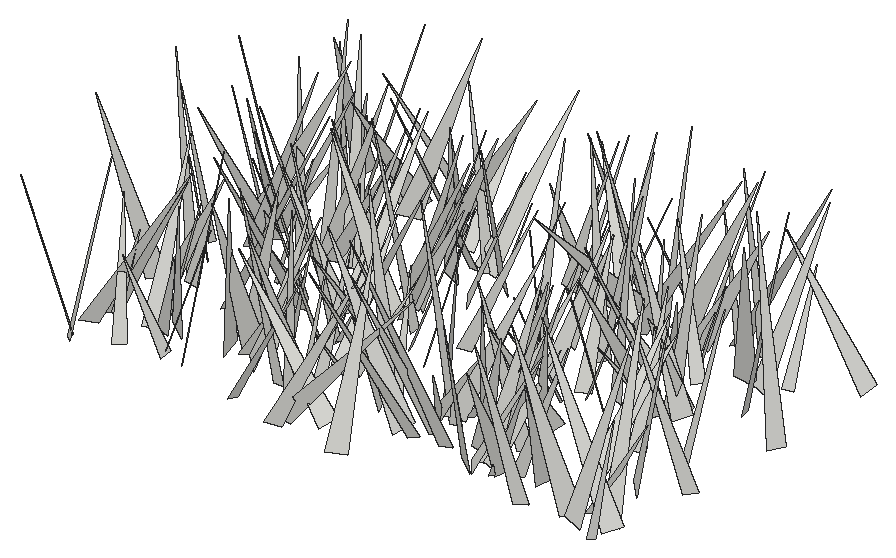
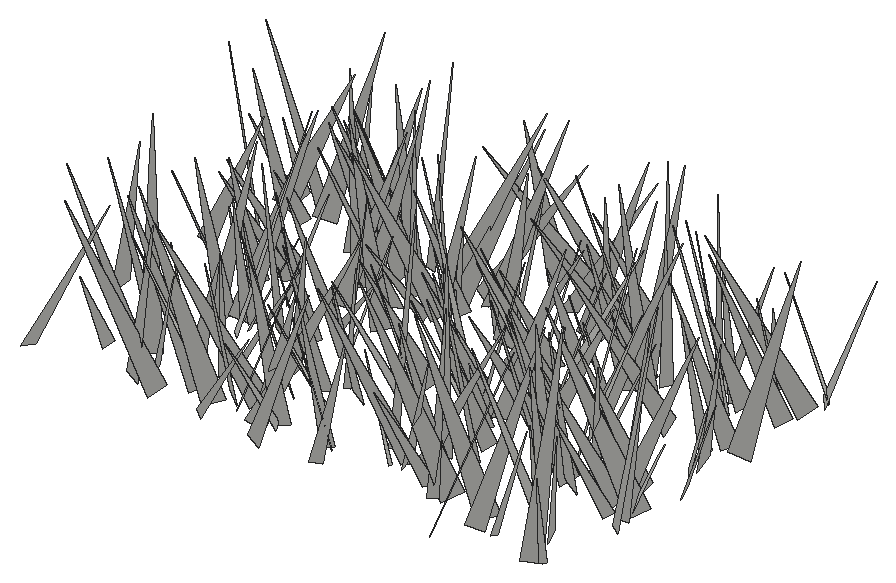
# SketchUp Ruby script. Lengths in inches.
U = 1.inch
M = Sketchup.active_model
def pt(a) = Geom::Point3d.new(a.map { |v| v * U })
def face(e, loops, mat)
  f = e.add_face(loops[0].map { |a| pt(a) })
  loops[1..].each { |l| e.add_face(l.map { |a| pt(a) }).erase! }
  f.material = f.back_material = mat if mat
  f
end
# faces: each face lists its corners as indices into pts; further lists are holes
def faces(e, pts, list, mat = nil) = list.each { |f| face(e, (f[0].is_a?(Array) ? f : [f]).map { |l| l.map { |i| pts[i] } }, mat) }
# xy, xz, yz: faces in a plane at the given z, y or x. An outline is a flat list of corners, or four numbers for a rectangle; further outlines are holes
def ring(l) = l.size == 4 ? [[l[0], l[1]], [l[2], l[1]], [l[2], l[3]], [l[0], l[3]]] : l.each_slice(2).to_a
def flat(e, list, mat, &to3) = list.each { |f| face(e, (f[0].is_a?(Array) ? f : [f]).map { |l| ring(l).map { |u, v| to3.(u, v) } }, mat) }
def xy(e, z, list, mat = nil) = flat(e, list, mat) { |x, y| [x, y, z] }
def xz(e, y, list, mat = nil) = flat(e, list, mat) { |x, z| [x, y, z] }
def yz(e, x, list, mat = nil) = flat(e, list, mat) { |y, z| [x, y, z] }
def lines(e, pts, list) = list.each { |a, b| e.add_line(pt(pts[a]), pt(pts[b])) }
# prism: a flat outline (further loops are holes) pulled along v
def prism(e, loops, v, mat = nil)
  f = face(e, loops, mat); d = Geom::Vector3d.new(v.map { |x| x * U })
  f.pushpull(f.normal.samedirection?(d) ? d.length : -d.length)
end
def box(e, o, s, mat = nil) = prism(e, [[o, [o[0] + s[0], o[1], o[2]], [o[0] + s[0], o[1] + s[1], o[2]], [o[0], o[1] + s[1], o[2]]]], [0, 0, s[2]], mat)
def at(x, y, z, deg = 0) = Geom::Transformation.translation(pt([x, y, z])) * Geom::Transformation.rotation(ORIGIN, Z_AXIS, deg.degrees)
def axes(o, x, y, z) = Geom::Transformation.new([*x, 0, *y, 0, *z, 0, *pt(o).to_a, 1])
def part(name) = M.definitions.add(name)
# library, detail: a bought-in or finely detailed component or shape, given as its bounding box
def library(name, o, s) = part(name).tap { |d| box(d.entities, o, s) }
def detail(e, o, s) = box(e.add_group.entities, o, s)
def put(e, d, t, mat = nil) = e.add_instance(d, t).tap { |i| i.material = mat if mat }
def group(e, t, mat = nil) = e.add_group.tap { |g| g.transformation = t; g.material = mat if mat }.entities
root = M.entities
c1 = part("fur_instance\#9")
p = [[0.8125,0,1.79],[0.67,-0.02,1.48],[0,-0.11,0],[0,0.11,0]]
faces(c1.entities,p,[[0,1,2,3]])
put(root,c1,axes([454.91,205.7,-21.66],[-4.61833,-3.74237,0.73758],[-3.79853,4.40694,-1.4242],[-0.34716,1.56584,5.77113]))
put(root,c1,axes([493.85,206.16,-21.66],[-0.12405,-5.8754,2.10648],[-6.00776,-0.4589,-1.63376],[-1.69244,2.05962,5.64504]))
put(root,c1,axes([479.56,203.79,-21.66],[-4.86903,5.31705,1.90275],[5.12727,5.21523,-1.45307],[2.36698,-0.35954,7.06166]))
put(root,c1,axes([487.54,207.98,-21.66],[-3.32814,-6.39102,1.50803],[-6.07577,3.63841,2.01068],[2.49085,0.3356,6.91945]))
put(root,c1,axes([490.22,208.89,-21.66],[5.08436,-3.96797,0.13679],[-3.71243,-4.83007,-2.12193],[-1.40762,-1.5937,6.0904]))
put(root,c1,axes([497.54,207.12,-21.66],[2.58278,-6.81445,2.81399],[-6.72051,-3.40212,-2.07037],[-3.03151,1.73634,6.98721]))
put(root,c1,axes([461.82,207.3,-21.66],[-4.35378,0.44066,1.23045],[0.84047,4.2213,1.46212],[1.0009,-1.62788,4.12453]))
put(root,c1,axes([476.5,206.75,-21.66],[-6.39943,2.86094,0.01202],[2.71801,6.07041,2.2137],[-0.89308,-2.0256,6.65111]))
put(root,c1,axes([473.63,204.27,-21.66],[5.89458,-2.32049,1.52507],[-2.76984,-5.16651,2.8446],[-0.1962,3.22166,5.6603]))
put(root,c1,axes([473.56,205.26,-21.66],[6.0984,-4.54505,0.22334],[-3.82324,-4.91501,4.37303],[2.46783,3.61705,6.22291]))
put(root,c1,axes([469.2,205.45,-21.66],[5.44463,0.12063,0.24069],[0.04962,-5.23956,1.50366],[-0.26462,1.49964,5.23426]))
put(root,c1,axes([500.63,205.45,-21.66],[-3.9364,0.91485,1.26316],[0.41585,3.92071,-1.54367],[1.50319,1.31107,3.73488]))
put(root,c1,axes([473.46,208.66,-21.66],[-0.04463,-6.97717,1.39975],[-6.92736,-0.27772,-1.60522],[-1.62845,1.37265,6.79015]))
put(root,c1,axes([493.23,209.51,-21.66],[5.19652,-2.78136,0.42044],[-2.54268,-5.02221,-1.79688],[-1.20313,-1.39929,5.61347]))
put(root,c1,axes([498.26,206.3,-21.66],[2.40948,7.1196,1.80641],[7.28749,-2.07931,-1.52526],[0.91887,-2.17835,7.35989]))
put(root,c1,axes([455.21,204.92,-21.66],[4.3588,4.87451,1.02077],[4.50794,-4.43827,1.9448],[-2.11691,0.58556,6.24322]))
put(root,c1,axes([482.32,208.84,-21.66],[-2.35699,-6.63901,0.53799],[-6.01099,1.87426,-3.2057],[-2.86948,1.52709,6.27339]))
put(root,c1,axes([461.04,208.54,-21.66],[5.75664,2.23558,0.62086],[2.31995,-5.52205,-1.62697],[0.03364,-1.74108,5.95732]))
put(root,c1,axes([501.0625,207.28,-21.66],[-3.57057,6.8988,1.02898],[6.50769,2.8788,3.28081],[-2.51043,-2.34953,7.04122]))
put(root,c1,axes([483.25,210.26,-21.66],[0.03934,-7.1777,0.79174],[-6.87762,-0.27857,-2.18369],[-2.20103,0.74216,6.83757]))
put(root,c1,axes([484.83,209.18,-21.66],[-3.02685,-7.70536,1.30124],[-7.48247,2.45538,-2.86554],[-2.25353,2.19686,7.76679]))
put(root,c1,axes([460.31,210.42,-21.66],[-2.5118,-6.70095,1.69222],[-6.07027,2.9998,2.86854],[3.30427,0.41708,6.55616]))
put(root,c1,axes([459.66,209.64,-21.66],[0.42063,-4.67833,0.35233],[-4.37367,-0.26302,1.72907],[1.69763,0.48155,4.36738]))
put(root,c1,axes([481.02,209.37,-21.66],[-7.69272,2.37823,1.5322],[2.71051,7.46743,2.01798],[0.8104,-2.40066,7.79498]))
put(root,c1,axes([487.1,210.29,-21.66],[1.41766,-6.83451,0.48866],[-6.53171,-1.19719,2.20513],[2.07029,0.90294,6.62252]))
put(root,c1,axes([487.97,208.14,-21.66],[4.83025,3.81866,0.07193],[3.65702,-4.5907,-1.86288],[1.10161,-1.50398,5.86882]))
put(root,c1,axes([458.41,206.45,-21.66],[-4.8792,2.06982,0.10093],[1.96371,4.70056,-1.46614],[0.66196,1.31208,5.09325]))
put(root,c1,axes([464.78,210.66,-21.66],[7.73874,0.04549,1.82687],[0.5794,-7.60007,-2.26513],[-1.73315,-2.33761,7.39995]))
put(root,c1,axes([498.41,208.22,-21.66],[4.05513,-1.76427,0.28786],[-1.75227,-3.78191,1.50543],[0.35366,1.49134,4.15818]))
put(root,c1,axes([472.51,206.64,-21.66],[5.53562,0.75174,0.06867],[0.66774,-5.11345,2.14935],[-0.35205,2.12143,5.1564]))
put(root,c1,axes([465.82,211.94,-21.66],[6.63906,-4.24471,1.17982],[-3.75911,-6.57064,-2.48644],[-2.29753,-1.51516,7.47745]))
put(root,c1,axes([455.8,209.32,-21.66],[1.53162,3.70831,1.75315],[4.01532,-0.97314,-1.44953],[0.83802,-2.1148,3.74116]))
put(root,c1,axes([454.82,207.59,-21.66],[6.90826,-2.9112,0.5406],[-2.88435,-6.30625,2.89882],[0.66922,2.87186,6.91346]))
put(root,c1,axes([472.45,207.48,-21.66],[-6.55431,0.09701,1.7896],[-0.34688,6.588,-1.62754],[1.75834,1.66126,6.34976]))
put(root,c1,axes([477.84,210.91,-21.66],[-4.12038,-2.11418,1.50488],[-1.47976,4.23386,1.89649],[2.13184,-1.14743,4.225]))
put(root,c1,axes([470.51,208.82,-21.66],[-3.32037,-5.8988,2.51801],[-6.36421,2.67847,-2.11746],[-0.7956,3.19234,6.42939]))
put(root,c1,axes([474.22,212.03,-21.66],[-2.58943,-3.13022,0.07236],[-2.65217,2.2427,2.10831],[1.66419,-1.2964,3.47253]))
put(root,c1,axes([463.49,207.03,-21.66],[5.66789,4.81372,1.80284],[4.22946,-5.89252,2.43659],[-2.92126,0.80836,7.02566]))
put(root,c1,axes([491.27,208.98,-21.66],[5.10289,-1.83511,1.25864],[-2.13691,-4.91957,1.49087],[-0.62081,1.84972,5.21387]))
put(root,c1,axes([482.33,211.77,-21.66],[3.64505,-0.39812,0.27738],[-0.20845,-3.18305,-1.82936],[-0.43816,-1.79764,3.17779]))
put(root,c1,axes([489.04,208.9,-21.66],[-0.29614,5.30233,1.4786],[4.87042,0.94241,-2.40408],[2.56516,-1.17721,4.73528]))
put(root,c1,axes([467.18,210.06,-21.66],[5.13352,5.29295,1.04527],[5.31008,-4.70157,-2.27141],[0.95446,-2.31104,7.01492]))
put(root,c1,axes([458.76,211.43,-21.66],[5.69332,3.04756,1.30745],[3.31373,-5.12843,-2.47574],[0.12746,-2.79687,5.96424]))
put(root,c1,axes([455.27,209.67,-21.66],[6.30652,-2.10429,0.15189],[-2.07978,-6.12031,1.56194],[0.35446,1.52876,6.46224]))
put(root,c1,axes([489.92,212.91,-21.66],[-0.39765,-7.51588,0.89638],[-7.02687,0.7002,2.75371],[2.81337,0.68655,7.00455]))
put(root,c1,axes([486.05,211.92,-21.66],[6.38697,0.74513,2.00431],[1.2691,-6.40204,-1.66407],[-1.72101,-1.95564,6.21124]))
put(root,c1,axes([500.6,207.55,-21.66],[0.70826,8.01559,0.32411],[7.89046,-0.75477,1.42384],[-1.44754,-0.19233,7.91985]))
put(root,c1,axes([489.875,208.25,-21.66],[7.02888,1.27959,1.54515],[0.73768,-6.88381,2.34499],[-1.86566,2.099,6.7486]))
put(root,c1,axes([481.875,211.4375,-21.66],[2.63596,-3.80697,0.02165],[-3.40971,-2.34911,2.07299],[1.69332,1.196,4.14053]))
put(root,c1,axes([488.5,209.21,-21.66],[6.0321,-2.57805,3.10449],[-3.62742,-5.91038,2.14001],[-1.76807,3.33038,6.20104]))
put(root,c1,axes([465.17,212.2,-21.66],[0.9927,-7.18833,2.00129],[-7.23058,-0.4281,2.04891],[1.84279,2.19257,6.96128]))
put(root,c1,axes([466.07,210.69,-21.66],[4.34648,-1.55951,0.20323],[-1.53377,-4.07129,1.56122],[0.34774,1.53551,4.34586]))
put(root,c1,axes([489.51,212.12,-21.66],[0.21483,-6.37799,2.26736],[-6.52313,-0.80094,-1.63496],[-1.80789,2.13204,6.16862]))
put(root,c1,axes([488.29,210.07,-21.66],[6.56769,-0.93589,1.93904],[-1.50422,-6.44796,1.98276],[-1.54048,2.30611,6.3308]))
put(root,c1,axes([498.67,212.66,-21.66],[5.37674,4.78999,2.15375],[5.23773,-5.117,-1.69543],[-0.38579,-2.71372,6.99849]))
put(root,c1,axes([489.21,215.83,-21.66],[4.98513,-4.06782,0.78587],[-3.3159,-4.65458,-3.05875],[-2.48386,-1.95039,5.66063]))
put(root,c1,axes([472.21,211.14,-21.66],[-4.0426,1.99311,1.15136],[1.52694,4.06338,-1.67276],[1.72237,1.07573,4.18533]))
put(root,c1,axes([471.03,211.07,-21.66],[1.74005,3.73475,0.21366],[3.48509,-1.70407,1.40429],[-1.35946,0.41179,3.87351]))
put(root,c1,axes([458.6875,209.61,-21.66],[-5.84983,3.65343,0.11485],[3.32744,5.4123,-2.68634],[1.51292,2.22277,6.35229]))
put(root,c1,axes([483.51,211.96,-21.66],[1.68916,7.29229,2.94864],[7.0223,-2.75681,2.79508],[-3.5439,-1.98689,6.94394]))
put(root,c1,axes([466.52,212.73,-21.66],[-0.20342,5.45726,1.92359],[5.57072,0.70526,-1.41173],[1.56492,-1.80117,5.27542]))
put(root,c1,axes([477.17,213,-21.66],[-0.80473,7.1427,2.6366],[7.51279,0.31449,1.44102],[-1.23607,-2.73867,7.04196]))
put(root,c1,axes([454.72,215.24,-21.66],[1.74253,-7.39949,2.19817],[-7.33714,-2.28781,-1.88496],[-2.39807,1.62304,7.36449]))
put(root,c1,axes([471.05,213.38,-21.66],[-6.43148,-3.95381,0.27263],[-3.76371,5.93049,-2.78112],[-1.24153,2.50351,7.01869]))
put(root,c1,axes([474.47,216.24,-21.66],[0.43766,-5.35462,0.13989],[-4.92597,-0.45748,-2.09965],[-2.10387,-0.04276,4.94519]))
put(root,c1,axes([478.31,211.9,-21.66],[-4.48023,1.71415,0.10108],[1.53614,4.12726,-1.90446],[0.76734,1.74596,4.4027]))
put(root,c1,axes([473.56,213.66,-21.66],[2.80072,3.68056,0.20092],[3.50306,-2.57922,-1.58339],[1.14693,-1.10998,4.34551]))
put(root,c1,axes([480,215.34,-21.66],[6.17791,2.14602,1.95241],[2.61385,-6.11017,-1.55482],[-1.25898,-2.15507,6.35252]))
put(root,c1,axes([456,214.62,-21.66],[4.35594,-4.3452,0.48537],[-4.22774,-4.01128,2.03138],[1.11472,1.7662,5.80763]))
put(root,c1,axes([502.04,214.58,-21.66],[-0.7555,-5.85213,2.53673],[-5.87032,-0.36099,-2.58111],[-2.49433,2.62211,5.30623]))
put(root,c1,axes([482.92,212.63,-21.66],[6.18283,-3.26103,2.17206],[-3.91127,-5.37775,3.05962],[-0.2327,3.74499,6.28493]))
put(root,c1,axes([484.88,216.63,-21.66],[3.43044,-6.71204,0.2285],[-6.5076,-3.25868,1.97581],[1.6598,1.09595,7.27431]))
put(root,c1,axes([486.01,213.59,-21.66],[1.82211,6.46965,0.85286],[6.26515,-1.48669,-2.10749],[1.8253,-1.35544,6.38239]))
put(root,c1,axes([483.59,213.57,-21.66],[3.8069,0.05751,0.20355],[-0.0416,-3.39391,1.73693],[-0.20739,1.73647,3.38805]))
put(root,c1,axes([465.04,218.09,-21.66],[-0.88458,-7.33954,0.10795],[-7.20369,0.84713,-1.43254],[-1.40973,0.27658,7.25253]))
put(root,c1,axes([457.01,216.09,-21.66],[1.41484,-4.55258,1.06253],[-4.54528,-1.07998,1.42506],[1.09333,1.40157,4.54939]))
put(root,c1,axes([467.33,214.15,-21.66],[3.33394,1.47543,1.26624],[0.9738,-3.44268,1.44745],[-1.68284,0.93087,3.34618]))
put(root,c1,axes([472.29,213.38,-21.66],[-2.9389,4.8588,0.20427],[4.55933,2.83593,-1.85926],[1.6918,0.79774,5.36547]))
put(root,c1,axes([494.95,213.39,-21.66],[-2.16647,5.60636,0.16983],[5.26617,2.09582,-2.00715],[1.93067,0.57445,5.66535]))
put(root,c1,axes([494.17,215.14,-21.66],[-1.05033,5.0969,0.69056],[4.61293,1.24522,-2.17458],[2.27512,-0.17172,4.72788]))
put(root,c1,axes([469.95,215.85,-21.66],[-6.83624,-2.0461,0.45627],[-2.08301,6.45462,-2.26447],[-0.23611,2.29788,6.76704]))
put(root,c1,axes([476.08,218.08,-21.66],[7.20484,3.15988,1.15153],[3.35999,-6.88107,-2.14053],[-0.14588,-2.42624,7.57051]))
put(root,c1,axes([492.64,217.48,-21.66],[-4.27144,-3.27285,0.83505],[-3.36103,3.98484,-1.57435],[-0.33515,1.75031,5.14569]))
put(root,c1,axes([493.46,221.62,-21.66],[3.75973,-6.87339,0.18092],[-6.4988,-3.61971,-2.46477],[-2.2454,-1.03249,7.43666]))
put(root,c1,axes([484.69,220.45,-21.66],[-2.93741,-3.09466,0.01129],[-2.71699,2.58635,2.03327],[1.48156,-1.39259,3.75115]))
put(root,c1,axes([461.02,214.95,-21.66],[7.74445,1.42991,0.81828],[1.0012,-7.20795,3.11989],[-1.30836,2.94814,7.231]))
put(root,c1,axes([462.92,220.02,-21.66],[-3.99864,-1.03805,0.42764],[-0.78188,3.71014,1.695],[0.80565,-1.55139,3.76744]))
put(root,c1,axes([470.14,216.41,-21.66],[7.35163,-0.33714,0.71191],[-0.54127,-7.01692,2.26646],[-0.57229,2.30568,7.00167]))
put(root,c1,axes([495.49,216.81,-21.66],[-4.4871,3.83069,1.41429],[3.5666,4.69982,-1.41404],[1.98841,0.2144,5.72789]))
put(root,c1,axes([467.85,219.39,-21.66],[-2.55985,4.83206,1.74885],[4.89019,1.69025,2.4878],[-1.579,-2.59892,4.86955]))
put(root,c1,axes([486.34,218.33,-21.66],[3.70498,4.05955,2.96614],[3.93602,-4.63444,1.42637],[-3.1282,-1.02317,5.30776]))
put(root,c1,axes([487.06,219.05,-21.66],[-2.6027,-3.00196,0.39616],[-2.70686,2.07255,-2.07851],[-1.35707,1.62343,3.38609]))
put(root,c1,axes([499.68,216.56,-21.66],[2.78013,5.13783,0.11647],[4.85085,-2.66723,1.86951],[-1.69707,0.79284,5.53456]))
put(root,c1,axes([464.61,219.31,-21.66],[-5.23852,-3.39609,0.6769],[-3.443,4.97658,-1.67721],[-0.37061,1.77027,6.01352]))
put(root,c1,axes([492.27,223.47,-21.66],[-6.0329,-5.73941,0.68236],[-5.34499,5.91535,2.49841],[2.19943,-1.36753,7.94322]))
put(root,c1,axes([455.95,219.24,-21.66],[-3.1769,-1.92196,0.83625],[-2.09296,2.82701,-1.45378],[-0.11299,1.67333,3.4166]))
put(root,c1,axes([487.82,221.19,-21.66],[5.19096,1.17327,0.15724],[1.14991,-4.82989,-1.92283],[0.28108,-1.90867,4.96239]))
put(root,c1,axes([456,217.59,-21.66],[-7.80069,-0.47128,0.71432],[-0.70737,7.23754,-2.94972],[0.48165,2.99651,7.23686]))
put(root,c1,axes([462.84,222.96,-21.66],[-6.10663,-5.12788,1.30944],[-4.81653,6.21333,1.86984],[2.19336,-0.63253,7.75176]))
put(root,c1,axes([470.64,221.17,-21.66],[-5.74656,4.30747,2.03787],[4.75581,5.38477,2.02895],[0.29923,-2.86007,6.88916]))
put(root,c1,axes([492,222.4,-21.66],[-3.24466,-1.65637,0.06319],[-1.44148,2.88818,1.68993],[0.81834,-1.47993,3.2273]))
put(root,c1,axes([474.39,218.39,-21.66],[4.68389,2.5085,0.46697],[2.25732,-4.52881,1.68637],[-1.1896,1.28326,5.03861]))
put(root,c1,axes([492.3,221.45,-21.66],[1.15805,-3.96128,0.43832],[-3.70743,-0.90324,1.63219],[1.46246,0.84697,3.79062]))
put(root,c1,axes([495.01,222.41,-21.66],[4.68158,-4.31782,3.21331],[-4.18207,-5.59908,-1.43065],[-3.3881,0.94493,6.20597]))
put(root,c1,axes([494.79,223.34,-21.66],[4.08531,-1.79648,1.28746],[-1.24322,-4.1049,-1.78292],[-1.82737,-1.22355,4.09124]))
put(root,c1,axes([473.0625,220.54,-21.66],[-7.26619,-2.16018,0.91047],[-2.32448,7.02333,-1.88745],[0.30351,2.07347,7.34176]))
put(root,c1,axes([468.41,218.49,-21.66],[6.47169,4.71895,0.84374],[4.29058,-6.33416,2.51645],[-2.13805,1.57262,7.60387]))
put(root,c1,axes([461.51,219.81,-21.66],[2.88186,3.44939,0.31018],[3.15851,-2.7832,1.60537],[-1.42067,0.8094,4.19835]))
put(root,c1,axes([457.41,224.5625,-21.66],[0.6668,-6.36542,0.43774],[-6.10772,-0.7641,-1.80742],[-1.84553,0.22889,6.13974]))
put(root,c1,axes([484.39,221.1,-21.66],[0.24671,6.36494,1.6516],[6.30189,0.24313,-1.87833],[1.87786,-1.65213,6.08648]))
put(root,c1,axes([477.34,220.6,-21.66],[5.30796,-1.91017,1.71118],[-2.50762,-4.68997,2.54311],[-0.53734,3.01775,5.03546]))
put(root,c1,axes([470.7,223.03,-21.66],[2.62599,-5.06265,0.78885],[-4.77605,-2.09765,2.43674],[1.85526,1.76578,5.15641]))
put(root,c1,axes([481.65,224.51,-21.66],[4.12034,-0.14152,0.59374],[0.17297,-3.61498,-2.06197],[-0.58535,-2.06437,3.57009]))
put(root,c1,axes([487.48,220.99,-21.66],[-4.32625,3.6169,1.13686],[3.35652,4.45591,-1.40339],[1.76301,0.39209,5.46158]))
put(root,c1,axes([454.46,221.61,-21.66],[-5.41168,-1.42657,0.35166],[-1.45652,5.03228,-1.99993],[-0.1932,2.0214,5.22701]))
put(root,c1,axes([493.19,221.17,-21.66],[-6.05732,0.47074,1.68041],[-0.07648,5.99257,-1.95441],[1.74342,1.89841,5.75265]))
put(root,c1,axes([471.32,221.46,-21.66],[6.28882,0.29269,0.74734],[0.08478,-6.11246,1.68051],[-0.79813,1.65699,6.06719]))
put(root,c1,axes([489.93,221.48,-21.66],[3.45024,7.01244,2.07893],[6.95776,-3.8555,1.45774],[-2.25516,-1.1667,7.67811]))
put(root,c1,axes([494.21,222.08,-21.66],[-6.74927,1.80081,2.69667],[1.18797,7.16726,-1.81295],[3.01723,1.2063,6.74602]))
put(root,c1,axes([462.65,224.625,-21.66],[4.53332,-3.78068,0.06575],[-3.6354,-4.32956,1.69931],[1.04008,1.34544,5.65304]))
put(root,c1,axes([455.38,227.19,-21.66],[-1.80775,-6.68688,0.47497],[-6.40102,1.86794,1.93536],[1.9917,-0.06601,6.65106]))
put(root,c1,axes([467.12,221.06,-21.66],[-4.67484,5.38464,0.57126],[4.73589,4.43174,-3.01759],[2.62527,1.59378,6.46085]))
put(root,c1,axes([479.14,222.34,-21.66],[4.7893,3.01055,0.30481],[2.77693,-4.59952,1.79634],[-1.20208,1.36921,5.36414]))
put(root,c1,axes([489.45,226.7,-21.66],[-4.59032,-0.23962,0.17171],[-0.16134,4.28449,1.66587],[0.24672,-1.65642,4.28408]))
put(root,c1,axes([456.87,222.81,-21.66],[6.5419,0.41912,1.71437],[-0.23349,-6.31856,2.43568],[-1.74935,2.41069,6.08602]))
put(root,c1,axes([502.66,223.11,-21.66],[-8.1921,1.36867,0.61461],[1.20152,8.02801,-1.8625],[0.89853,1.74336,8.09413]))
put(root,c1,axes([463.77,225.21,-21.66],[3.63408,5.21962,1.38175],[5.32326,-3.18476,-1.96987],[0.90365,-2.23003,6.04736]))
put(root,c1,axes([468.93,224.9,-21.66],[5.6454,-1.61471,0.55375],[-1.70236,-5.46688,1.41409],[-0.12614,1.5134,5.69896]))
put(root,c1,axes([482.48,225.71,-21.66],[0.05129,-4.93553,2.34933],[-4.99892,0.90807,2.01684],[2.21125,2.16734,4.50493]))
put(root,c1,axes([468.37,226.93,-21.66],[5.01746,5.30698,2.27397],[5.71554,-4.13917,-2.95123],[0.81705,-3.63499,6.68051]))
put(root,c1,axes([473.91,229.1875,-21.66],[-3.7888,-7.35051,1.42507],[-6.56657,4.02946,3.32556],[3.59735,-0.38635,7.57137]))
put(root,c1,axes([471.67,223.03,-21.66],[4.6203,4.92142,0.32663],[4.69042,-4.52255,1.79463],[-1.52544,1.00021,6.50745]))
put(root,c1,axes([473.32,225.98,-21.66],[5.31801,3.62577,0.57345],[3.65614,-5.14142,-1.39812],[0.32822,-1.47507,6.28273]))
put(root,c1,axes([454.96,228.49,-21.66],[-4.90749,-6.3294,1.61985],[-6.13533,5.16095,1.5783],[2.24565,0.26836,7.85199]))
put(root,c1,axes([495.2,229.125,-21.66],[1.43301,-8.2393,0.15598],[-8.02359,-1.35888,1.93375],[1.87948,0.48092,8.13635]))
put(root,c1,axes([461.71,225.13,-21.66],[6.69974,-1.69034,1.74311],[-2.11177,-6.58131,1.73465],[-1.19837,2.1474,6.68841]))
put(root,c1,axes([470.45,227.77,-21.66],[-1.45623,-6.82166,1.9418],[-6.84757,1.86878,1.42991],[1.84835,1.54881,6.82723]))
put(root,c1,axes([460.1,224.35,-21.66],[-6.71472,0.14595,1.05093],[-0.21339,6.41005,-2.25365],[1.03933,2.25902,6.32691]))
put(root,c1,axes([455.04,225.82,-21.66],[6.5519,-4.81181,0.9912],[-4.80718,-5.93833,2.94799],[1.01342,2.94042,7.57563]))
put(root,c1,axes([464.29,224.91,-21.66],[-5.1152,1.11044,1.16629],[0.73583,5.06638,-1.59654],[1.43244,1.36283,4.98492]))
put(root,c1,axes([489.3,228.51,-21.66],[-0.15941,-4.26775,0.08772],[-3.87813,0.18147,1.78158],[1.78369,0.01316,3.88138]))
put(root,c1,axes([455.64,225.9,-21.66],[-4.45593,-2.02584,0.38216],[-1.95722,3.87117,-2.29973],[-0.64758,2.23951,4.32095]))
put(root,c1,axes([460.95,229.875,-21.66],[-1.84691,-6.18778,0.26193],[-5.9057,1.84189,1.87043],[1.86547,-0.29517,6.18071]))
put(root,c1,axes([464.13,224.59,-21.66],[0.27633,8.1596,0.76138],[7.93766,-0.45592,2.00518],[-2.0377,-0.66947,7.91421]))
put(root,c1,axes([457.15,225.5,-21.66],[6.04009,-0.71684,0.90558],[-1.00409,-5.64184,2.23115],[-0.57074,2.3393,5.65849]))
put(root,c1,axes([485.76,225.29,-21.66],[-7.72963,0.57294,0.92033],[0.30078,7.49944,-2.14251],[1.04153,2.08628,7.44883]))
put(root,c1,axes([497.92,225.62,-21.66],[6.4621,3.38539,1.99868],[3.00841,-6.73382,1.67909],[-2.53082,0.63956,7.09931]))
put(root,c1,axes([483.41,232.52,-21.66],[5.32765,-5.22538,0.29084],[-4.03169,-4.36253,-4.52625],[-3.33686,-3.07194,5.93309]))
put(root,c1,axes([456.56,227.23,-21.66],[3.29977,-2.51906,0.3221],[-2.3698,-2.86445,1.87534],[0.91296,1.66948,3.70368]))
put(root,c1,axes([480.27,225.05,-21.66],[2.16067,6.65454,0.44246],[6.23565,-2.18071,2.34697],[-2.36543,0.32979,6.59114]))
put(root,c1,axes([461.14,225.73,-21.66],[2.8075,7.47142,1.47372],[7.21104,-3.11318,2.04573],[-2.44844,-0.60171,7.71486]))
put(root,c1,axes([491.26,229.15,-21.66],[3.99613,2.0991,0.80323],[2.24013,-3.58697,-1.77087],[0.18236,-1.93595,4.15203]))
put(root,c1,axes([492.84,226.86,-21.66],[-1.19348,5.65379,0.3473],[5.3271,0.99964,2.033],[-1.92561,-0.73875,5.40894]))
put(root,c1,axes([470.83,229.78,-21.66],[-3.56669,-5.90918,0.59479],[-5.71236,3.22345,-2.22975],[-1.62517,1.63841,6.53207]))
put(root,c1,axes([484.51,227.16,-21.66],[4.61652,6.22378,1.13894],[6.03614,-4.75491,1.51682],[-1.89675,0.0163,7.59914]))
put(root,c1,axes([480.61,227.84,-21.66],[3.00596,2.69315,0.13963],[2.45938,-2.82346,1.51258],[-1.10635,1.04086,3.74179]))
put(root,c1,axes([467.49,232.86,-21.66],[-1.30326,-6.4856,0.41929],[-6.05179,1.36694,2.33336],[2.36951,-0.07596,6.19006]))
put(root,c1,axes([462.64,234.33,-21.66],[6.08431,-4.17162,0.61258],[-3.3903,-5.47976,-3.64343],[-2.50671,-2.71408,6.41457]))
put(root,c1,axes([472.63,231.1,-21.66],[3.70621,1.73352,0.50221],[1.78343,-3.34171,-1.62653],[0.27688,-1.67963,3.75439]))
put(root,c1,axes([489.52,231,-21.66],[2.95462,-6.48005,1.02046],[-5.97059,-2.19282,3.36242],[2.71745,2.2277,6.27814]))
put(root,c1,axes([496.72,228.75,-21.66],[1.72672,7.47142,1.23195],[7.48463,-1.49226,-1.44043],[1.14896,-1.50745,7.53186]))
put(root,c1,axes([467.25,231.39,-21.66],[3.81653,-4.78014,0.36891],[-4.62204,-3.54318,1.90641],[1.2738,1.46558,5.81217]))
put(root,c1,axes([482,231.32,-21.66],[1.0853,-7.02468,2.48253],[-7.23303,-0.3918,2.05344],[1.78669,2.68091,6.80495]))
put(root,c1,axes([486.08,230.7,-21.66],[-6.99068,-2.50094,0.47101],[-2.54423,6.83653,-1.46112],[-0.05835,1.53405,7.27938]))
put(root,c1,axes([477.54,231.79,-21.66],[1.22983,-5.08709,1.30795],[-5.046,-0.77126,1.74491],[1.45845,1.62123,4.93419]))
put(root,c1,axes([485.17,229.74,-21.66],[7.21653,-2.33327,0.39687],[-2.31249,-6.67999,2.77668],[0.50399,2.75925,7.05779]))
put(root,c1,axes([480.72,227.86,-21.66],[4.07419,5.57288,0.07978],[5.18286,-3.82462,2.48447],[-2.04971,1.40628,6.44076]))
put(root,c1,axes([484.37,229.99,-21.66],[-3.04335,5.85133,0.32291],[5.70958,2.87864,1.64877],[-1.32023,-1.03909,6.38604]))
put(root,c1,axes([487.54,231.83,-21.66],[4.40599,-6.63506,1.39046],[-6.52465,-3.70025,3.01783],[1.84021,2.76664,7.37085]))
put(root,c1,axes([466.51,231.91,-21.66],[6.17977,-5.38552,0.13557],[-5.06059,-5.73249,2.95646],[1.84733,2.31224,7.64543]))
put(root,c1,axes([477.4,231.71,-21.66],[5.01329,4.55618,1.17415],[4.70331,-4.80639,-1.43108],[0.12753,-1.84671,6.62147]))
put(root,c1,axes([471.96,230.02,-21.66],[-6.70082,0.16595,0.10129],[0.12128,6.29761,-2.29436],[0.15195,2.29157,6.29797]))
put(root,c1,axes([490.59,229.35,-21.66],[4.99959,5.18328,0.38062],[5.01525,-4.9501,1.53324],[-1.36326,0.79826,7.03643]))
put(root,c1,axes([498.22,230,-21.66],[-3.90191,2.21296,0.38649],[1.88444,3.64598,-1.85127],[1.22289,1.44261,4.08594]))
put(root,c1,axes([456.65,235.62,-21.66],[7.11754,-4.23376,0.53848],[-3.90576,-6.88369,-2.49681],[-1.7204,-1.88792,7.89621]))
put(root,c1,axes([471.64,230.06,-21.66],[-0.75445,7.6495,1.46212],[7.18414,1.25072,-2.83648],[3.00677,-1.06897,7.14412]))
put(root,c1,axes([502.54,233.42,-21.66],[-6.59727,0.97904,0.29915],[1.02311,6.37288,1.70633],[0.03533,-1.73199,6.44755]))
put(root,c1,axes([476.84,234.03,-21.66],[3.36953,-3.09183,0.80409],[-2.80421,-3.42236,-1.4084],[-1.53048,-0.53643,4.35081]))
put(root,c1,axes([493.36,230.92,-21.66],[-5.59441,-0.96055,0.72122],[-1.15543,5.24244,-1.98041],[0.32833,2.08191,5.31959]))
put(root,c1,axes([460.2,230.33,-21.66],[6.70956,3.50603,1.11128],[3.28027,-6.75003,1.49074],[-1.66343,0.8308,7.42214]))
put(root,c1,axes([460.97,234.26,-21.66],[-3.68775,-0.43694,1.2324],[0.03671,3.65173,1.40455],[1.30705,-1.33536,3.43768]))
put(root,c1,axes([494.14,232.52,-21.66],[1.80379,6.11401,2.80003],[6.29213,-2.55743,1.53087],[-2.37284,-2.13386,6.18799]))
put(root,c1,axes([486.97,230.375,-21.66],[3.53249,6.50702,1.2231],[6.07163,-3.73652,2.34297],[-2.64057,0.11331,7.02355]))
put(root,c1,axes([487.37,233.67,-21.66],[-2.45268,-3.25533,0.28731],[-3.08329,2.18606,-1.55237],[-1.08306,1.14864,3.76868]))
put(root,c1,axes([457.76,232.04,-21.66],[-5.24858,-0.93793,1.2858],[-1.33069,5.01688,-1.77222],[0.87308,2.00792,5.02857]))
put(root,c1,axes([482.15,231.6,-21.66],[3.84867,2.11329,0.22175],[1.92609,-3.66331,1.48248],[-0.8974,1.20066,4.13285]))
put(root,c1,axes([482.04,234.34,-21.66],[-2.37076,-5.83706,1.32394],[-5.9146,2.06646,-1.48049],[-0.91737,1.76156,6.12372]))
put(root,c1,axes([462.75,232.6875,-21.66],[5.54256,-5.39998,2.31392],[-5.86744,-4.92827,2.55329],[0.29519,3.43313,7.30483]))
put(root,c1,axes([464.42,236.95,-21.66],[-5.86145,-3.99032,0.23805],[-3.68658,5.55942,2.41617],[1.54546,-1.87245,6.66644]))
put(root,c1,axes([468.73,231.58,-21.66],[-1.68385,4.77561,0.18208],[4.53538,1.65768,-1.53538],[1.50664,0.34725,4.82539]))
put(root,c1,axes([456.03,235.27,-21.66],[-0.42992,-4.68733,0.89248],[-4.33891,0.75688,1.88505],[1.98531,0.63912,4.31306]))
put(root,c1,axes([491.55,232.99,-21.66],[7.5928,-1.32868,0.07278],[-1.31152,-7.40102,1.71058],[0.22497,1.69728,7.51598]))
